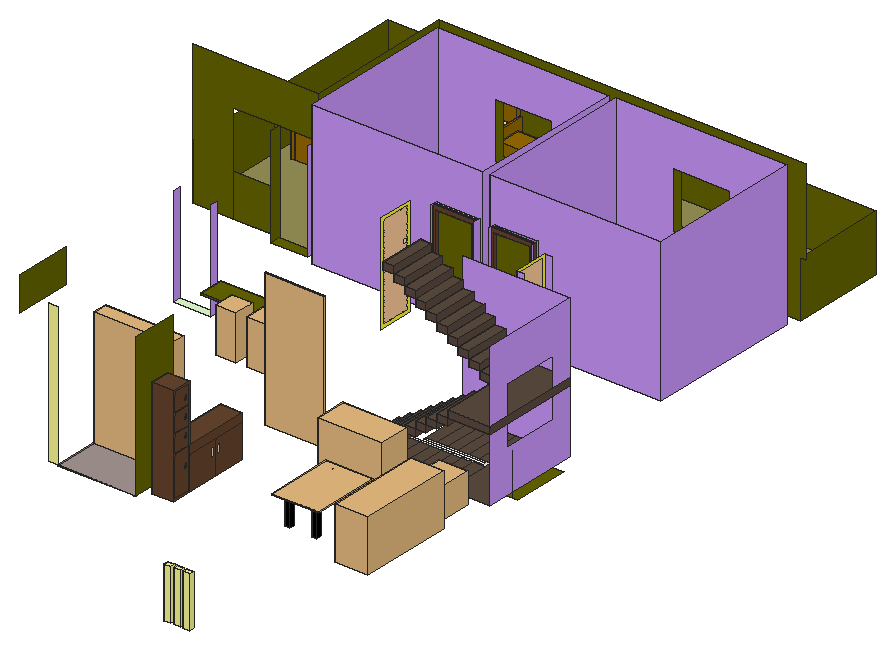
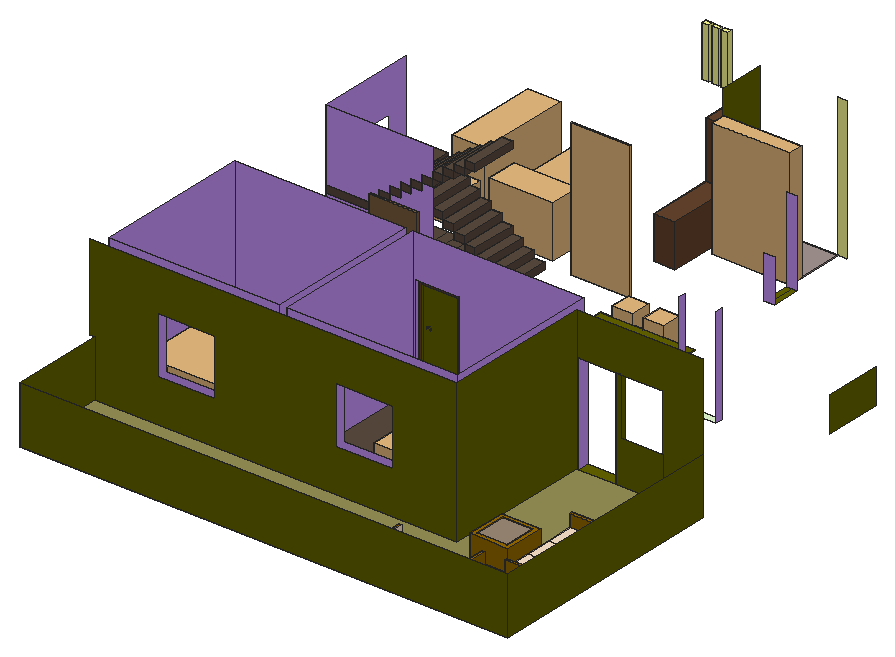
# SketchUp Ruby script. Lengths in inches.
U = 1.inch
M = Sketchup.active_model
def pt(a) = Geom::Point3d.new(a.map { |v| v * U })
def face(e, loops, mat)
  f = e.add_face(loops[0].map { |a| pt(a) })
  loops[1..].each { |l| e.add_face(l.map { |a| pt(a) }).erase! }
  f.material = f.back_material = mat if mat
  f
end
# faces: each face lists its corners as indices into pts; further lists are holes
def faces(e, pts, list, mat = nil) = list.each { |f| face(e, (f[0].is_a?(Array) ? f : [f]).map { |l| l.map { |i| pts[i] } }, mat) }
# xy, xz, yz: faces in a plane at the given z, y or x. An outline is a flat list of corners, or four numbers for a rectangle; further outlines are holes
def ring(l) = l.size == 4 ? [[l[0], l[1]], [l[2], l[1]], [l[2], l[3]], [l[0], l[3]]] : l.each_slice(2).to_a
def flat(e, list, mat, &to3) = list.each { |f| face(e, (f[0].is_a?(Array) ? f : [f]).map { |l| ring(l).map { |u, v| to3.(u, v) } }, mat) }
def xy(e, z, list, mat = nil) = flat(e, list, mat) { |x, y| [x, y, z] }
def xz(e, y, list, mat = nil) = flat(e, list, mat) { |x, z| [x, y, z] }
def yz(e, x, list, mat = nil) = flat(e, list, mat) { |y, z| [x, y, z] }
def lines(e, pts, list) = list.each { |a, b| e.add_line(pt(pts[a]), pt(pts[b])) }
# prism: a flat outline (further loops are holes) pulled along v
def prism(e, loops, v, mat = nil)
  f = face(e, loops, mat); d = Geom::Vector3d.new(v.map { |x| x * U })
  f.pushpull(f.normal.samedirection?(d) ? d.length : -d.length)
end
def box(e, o, s, mat = nil) = prism(e, [[o, [o[0] + s[0], o[1], o[2]], [o[0] + s[0], o[1] + s[1], o[2]], [o[0], o[1] + s[1], o[2]]]], [0, 0, s[2]], mat)
def at(x, y, z, deg = 0) = Geom::Transformation.translation(pt([x, y, z])) * Geom::Transformation.rotation(ORIGIN, Z_AXIS, deg.degrees)
def axes(o, x, y, z) = Geom::Transformation.new([*x, 0, *y, 0, *z, 0, *pt(o).to_a, 1])
def part(name) = M.definitions.add(name)
# library, detail: a bought-in or finely detailed component or shape, given as its bounding box
def library(name, o, s) = part(name).tap { |d| box(d.entities, o, s) }
def detail(e, o, s) = box(e.add_group.entities, o, s)
def put(e, d, t, mat = nil) = e.add_instance(d, t).tap { |i| i.material = mat if mat }
def group(e, t, mat = nil) = e.add_group.tap { |g| g.transformation = t; g.material = mat if mat }.entities
root = M.entities
M.materials.add("C01_Vanilla_Cream").color = [255, 230, 206]
M.materials.add("C02_Golden_Beige").color = [255, 205, 155]
M.materials.add("D07_Ochre_Flame").color = [153, 107, 0]
M.materials.add("E01_Mint_Frost").color = [255, 255, 204]
M.materials.add("E02_Pale_Lime").color = [255, 255, 153]
M.materials.add("E04_Green_Bloom").color = [255, 255, 49]
M.materials.add("E08_Lime_Depth").color = [102, 102, 0]
M.materials.add("Glass_Sky Reflection_01").color = [126, 138, 183]
M.materials["Glass_Sky Reflection_01"].alpha = 0.25
M.materials.add("J02_Lavender_Veil").color = [204, 153, 255]
M.materials.add("M09_Shadow_Night").color = [0, 0, 0]
M.materials.add("Marble_01_1K").color = [230, 255, 211]
M.materials.add("Marble_03_1K").color = [175, 182, 201]
M.materials.add("Marble_06_1K").color = [165, 150, 147]
M.materials.add("Marble_07_1K").color = [36, 34, 36]
M.materials.add("Marble_20_1K").color = [172, 173, 182]
M.materials.add("Metal_06_1K").color = [238, 236, 231]
M.materials.add("Plaster_02_1K").color = [157, 140, 119]
M.materials.add("Plywood_01_1K").color = [125, 96, 64]
M.materials.add("Soil_04_1K").color = [152, 146, 88]
M.materials.add("Wood_Floor_12_1K").color = [92, 75, 65]
M.materials.add("Wood_Veneer_15_1K").color = [103, 69, 45]
c1 = part("Group\#9")
box(c1.entities,[0,0,0],[0.75,3.75,0.1875],"Metal_06_1K")
c2 = part("Group\#2")
xy(c2.entities,0,[[0,-16.81,18.0625,0],[0,0,18.0625,55.25]],"Wood_Veneer_15_1K")
xy(c2.entities,36,[[0,0,18.0625,55.25]],"Wood_Veneer_15_1K")
xy(c2.entities,84,[[0,-16.81,18.0625,0]],"Wood_Veneer_15_1K")
xz(c2.entities,-16.81,[[0,0,18.0625,84]],"Wood_Veneer_15_1K")
xz(c2.entities,0,[[0,0,18.0625,36],[0,36,18.0625,84]],"Wood_Veneer_15_1K")
xz(c2.entities,55.25,[[0,0,18.0625,36]],"Wood_Veneer_15_1K")
yz(c2.entities,0,[[-16.81,0,0,84],[0,0,55.25,36]],"Wood_Veneer_15_1K")
yz(c2.entities,18.0625,[[[-16.81,0,0,84],[-14.81,2,-2,82]],[0,0,27.625,27.91],[27.625,0,55.25,27.91],[-14.81,2,-2,35],[0,27.91,55.25,36],
  [-14.81,35,-2,36],[-14.81,36,-2,50.3125],[-14.81,50.3125,-2,51.3125],[-14.81,51.3125,-2,65.85],[-14.81,65.85,-2,66.85],
  [-14.81,66.85,-2,82]],"Wood_Veneer_15_1K")
g1 = group(c2.entities,at(18.0625,23.18,16.77))
box(g1,[0,0,0],[0.2,1.5,6.25],"Metal_06_1K")
g2 = group(c2.entities,at(18.0625,29.74,16.77))
box(g2,[0,0,0],[0.2,1.5,6.25],"Metal_06_1K")
put(c2.entities,c1,axes([18.0625,-4.49,72.03],[0,1,0],[0,0,1],[1,0,0]))
put(c2.entities,c1,axes([18.0625,-4.49,57.4],[0,1,0],[0,0,1],[1,0,0]))
put(c2.entities,c1,axes([18.0625,-4.49,42.9],[0,1,0],[0,0,1],[1,0,0]))
put(c2.entities,c1,axes([18.0625,-4.49,20.71],[0,1,0],[0,0,1],[1,0,0]))
c3 = part("Group\#51")
xy(c3.entities,0,[[0,39,81,39,81,45,27,45,27,43,79,43,79,41,0,41]],"Metal_06_1K")
xy(c3.entities,0,[[0,0,9,39],[9,0,18,39],[18,0,27,39],[27,0,36,39],[36,0,45,39],
  [45,0,54,39],[54,0,63,39],[63,0,72,39],[72,0,81,39],[81,0,117,84],
  [27,45,36,84],[36,45,45,84],[45,45,54,84],[54,45,63,84],[63,45,72,84],
  [72,45,81,84]],"Wood_Floor_12_1K")
c4 = part("Group\#70")
box(c4.entities,[0,0,0],[9,39,6],"Wood_Floor_12_1K")
c5 = part("Group\#50")
xy(c5.entities,0,[[0,39,81,39,81,45,27,45,27,43,79,43,79,41,0,41]],"Metal_06_1K")
xy(c5.entities,0,[[9,0,18,39],[18,0,27,39],[27,0,36,39],[36,0,45,39],[45,0,54,39],
  [54,0,63,39],[63,0,72,39],[72,0,81,39],[81,0,117,84],[27,45,36,84],
  [36,45,45,84],[45,45,54,84],[54,45,63,84],[63,45,72,84],[72,45,81,84]],"Wood_Floor_12_1K")
put(c5.entities,c4,at(0,0,0))
put(c5.entities,c4,at(9,0,6))
put(c5.entities,c4,at(18,0,12))
put(c5.entities,c4,at(27,0,18))
put(c5.entities,c4,at(36,0,24))
put(c5.entities,c4,at(45,0,30))
put(c5.entities,c4,at(54,0,36))
put(c5.entities,c4,at(63,0,42))
put(c5.entities,c4,at(72,0,48))
g3 = group(c5.entities,at(81,0,54))
box(g3,[0,0,0],[36,84,6],"Wood_Floor_12_1K")
put(c5.entities,c4,at(72,45,60))
put(c5.entities,c4,at(63,45,66))
put(c5.entities,c4,at(54,45,72))
put(c5.entities,c4,at(45,45,78))
put(c5.entities,c4,at(36,45,84))
put(c5.entities,c4,at(27,45,90))
put(c5.entities,c4,at(18,45,96))
put(c5.entities,c4,at(9,45,102))
put(c5.entities,c4,at(0,45,108))
put(c5.entities,c4,at(-9,45,114))
c6 = part("Group\#41")
xy(c6.entities,0,[[[0,0,32.5625,34],[3.65,3.65,28.91,30.35]]],"D07_Ochre_Flame")
xy(c6.entities,18.3125,[[[0,0,32.5625,34],[3.65,3.65,28.91,30.35]]],"D07_Ochre_Flame")
xy(c6.entities,18.3125,[[3.65,3.65,28.91,30.35]],"Plaster_02_1K")
xz(c6.entities,0,[[0,0,32.5625,18.3125]],"D07_Ochre_Flame")
xz(c6.entities,3.65,[[3.65,0,28.91,18.3125]],"D07_Ochre_Flame")
xz(c6.entities,30.35,[[3.65,0,28.91,18.3125]],"D07_Ochre_Flame")
xz(c6.entities,34,[[0,0,32.5625,18.3125]],"D07_Ochre_Flame")
yz(c6.entities,0,[[0,0,34,18.3125]],"D07_Ochre_Flame")
yz(c6.entities,3.65,[[3.65,0,30.35,18.3125]],"D07_Ochre_Flame")
yz(c6.entities,28.91,[[3.65,0,30.35,18.3125]],"D07_Ochre_Flame")
yz(c6.entities,32.5625,[[0,0,34,18.3125]],"D07_Ochre_Flame")
c7 = library("Group\#27",[0,0,0],[94.3125,62.5,20])
c8 = part("Group\#17")
box(c8.entities,[0,0,0],[4,4,24])
c9 = part("Group\#16")
box(c9.entities,[0,0,0],[4,4,24])
c10 = part("Group\#29")
box(c10.entities,[0,0,0],[20.5,20.5,18],"Wood_Veneer_15_1K")
c11 = part("Group\#47")
box(c11.entities,[0,0,0],[65.6875,38.91,0.4375],"Marble_06_1K")
c12 = part("Group\#12")
detail(c12.entities,[-3,0,0],[54,27,43.625])
c13 = part("Group\#11")
detail(c13.entities,[0,0,0],[24,24,25.375])
c14 = part("Group\#10")
detail(c14.entities,[0,-4,0],[28,80,43.625])
c15 = part("Group\#14")
box(c15.entities,[0,0,0],[4,4,24])
c16 = part("Group\#15")
box(c16.entities,[0,0,0],[4,4,24])
c17 = part("Group\#38")
xy(c17.entities,0,[[67.3125,0,69.625,27.1875],[-2.33,24.1875,67.3125,27.1875]],"D07_Ochre_Flame")
xy(c17.entities,18.3125,[[0,0,22.82,24.1875],[22.82,0,45.07,24.1875],[45.07,0,67.3125,24.1875]],"C01_Vanilla_Cream")
xy(c17.entities,24.5625,[[67.3125,0,69.625,27.1875]],"D07_Ochre_Flame")
xy(c17.entities,28.6875,[[-2.33,0,0,24.1875]],"D07_Ochre_Flame")
xy(c17.entities,33.375,[[-2.33,24.1875,67.3125,27.1875]],"D07_Ochre_Flame")
xz(c17.entities,0,[[0,0,22.82,18.3125],[22.82,0,45.07,18.3125],[45.07,0,67.3125,18.3125]],"C01_Vanilla_Cream")
xz(c17.entities,0,[[-2.33,0,0,28.6875],[67.3125,0,69.625,24.5625]],"D07_Ochre_Flame")
xz(c17.entities,24.1875,[[-2.33,0,67.3125,0,67.3125,18.3125,0,18.3125,0,28.6875,-2.33,28.6875],[0,18.3125,22.82,33.375],[22.82,18.3125,45.07,33.375],[45.07,18.3125,67.3125,33.375],[-2.33,28.6875,0,33.375]],"D07_Ochre_Flame")
xz(c17.entities,27.1875,[[-2.33,0,67.3125,33.375],[67.3125,0,69.625,24.5625]],"D07_Ochre_Flame")
yz(c17.entities,-2.33,[[0,0,24.1875,28.6875],[24.1875,0,27.1875,33.375]],"D07_Ochre_Flame")
yz(c17.entities,0,[[0,18.3125,24.1875,28.6875]],"D07_Ochre_Flame")
yz(c17.entities,67.3125,[[0,0,24.1875,18.3125],[0,18.3125,24.1875,24.5625]],"C01_Vanilla_Cream")
yz(c17.entities,67.3125,[[24.1875,0,27.1875,24.5625],[24.1875,24.5625,27.1875,33.375]],"D07_Ochre_Flame")
yz(c17.entities,69.625,[[0,0,27.1875,24.5625]],"D07_Ochre_Flame")
c18 = part("Group\#43")
box(c18.entities,[0,0,0],[1,4.5625,0.25],"Metal_06_1K")
c19 = part("Group\#42")
xy(c19.entities,0,[[0,-1.93,40.35,0],[0,0,40.35,21.25]],"Plywood_01_1K")
xy(c19.entities,25.125,[[0,0,40.35,21.25]],"Marble_07_1K")
xy(c19.entities,25.1875,[[20.85,8.75,21.39,8.86,21.89,9.11,22.3,9.47,22.61,9.94,22.79,10.46,22.82,11.01,22.71,11.56,22.47,12.06,22.1,12.47,21.64,12.78,21.11,12.96,20.56,12.99,20.01,12.88,19.52,12.63,19.1,12.27,18.79,11.81,18.62,11.28,18.58,10.73,18.69,10.18,18.9375,9.69,19.31,9.27,19.77,8.96,20.29,8.79]],"M09_Shadow_Night")
xy(c19.entities,25.1875,[[[8.8,4,31.8,17.68],[20.85,8.75,20.29,8.79,19.77,8.96,19.31,9.27,18.9375,9.69,18.69,10.18,18.58,10.73,18.62,11.28,18.79,11.81,19.1,12.27,19.52,12.63,20.01,12.88,20.56,12.99,21.11,12.96,21.64,12.78,22.1,12.47,22.47,12.06,22.71,11.56,22.82,11.01,22.79,10.46,22.61,9.94,22.3,9.47,21.89,9.11,21.39,8.86]]],"Marble_07_1K")
xy(c19.entities,26,[[0,-1.93,40.35,0]],"Plywood_01_1K")
xy(c19.entities,26.5625,[[[0,0,40.35,21.25],[8.8,4,31.8,17.68]]],"Marble_07_1K")
xy(c19.entities,71.66,[[0,-1.93,40.35,0]],"Plywood_01_1K")
xz(c19.entities,-1.93,[[0,0,40.35,26],[0,26,40.35,71.66]],"Plywood_01_1K")
xz(c19.entities,0,[[0,25.125,40.35,26],[0,26,40.35,26.5625]],"Marble_07_1K")
xz(c19.entities,0,[[0,0,40.35,25.125],[0,26.5625,40.35,71.66]],"Plywood_01_1K")
xz(c19.entities,4,[[8.8,25.1875,31.8,26.5625]],"Marble_07_1K")
xz(c19.entities,17.68,[[8.8,25.1875,31.8,26.5625]],"Marble_07_1K")
xz(c19.entities,21.25,[[0,25.125,40.35,26.5625]],"Marble_07_1K")
xz(c19.entities,21.25,[[0,0,20.17,21],[20.17,0,40.35,21],[0,21,40.35,25.125]],"Plywood_01_1K")
yz(c19.entities,0,[[0,25.125,21.25,26.5625]],"Marble_07_1K")
yz(c19.entities,0,[[-1.93,0,0,26],[0,0,21.25,25.125],[-1.93,26,0,71.66]],"Plywood_01_1K")
yz(c19.entities,8.8,[[4,25.1875,17.68,26.5625]],"Marble_07_1K")
yz(c19.entities,31.8,[[4,25.1875,17.68,26.5625]],"Marble_07_1K")
yz(c19.entities,40.35,[[0,25.125,21.25,26.5625]],"Marble_07_1K")
yz(c19.entities,40.35,[[-1.93,0,0,26],[0,0,21.25,25.125],[-1.93,26,0,71.66]],"Plywood_01_1K")
put(c19.entities,c18,axes([22.63,21.25,13.17],[-1,0,0],[0,0,1],[0,1,0]))
put(c19.entities,c18,axes([18.69,21.25,13.17],[-1,0,0],[0,0,1],[0,1,0]))
put(c19.entities,c18,axes([22.61,21.25,24.2],[0,0,-1],[-1,0,0],[0,1,0]))
c20 = part("Group\#40")
box(c20.entities,[0,4,0],[19.9375,19.25,18.3125],"D07_Ochre_Flame")
c21 = library("Group\#36",[0,0,0],[17.25,17.25,38])
c22 = library("Group\#54",[0,-12,0],[65.6875,12,119.5625])
c23 = part("Group\#61")
prism(c23.entities,[[[0.51,0.51,0],[0.23,0.875,0],[0.06,1.3,0],[0,1.75,0],[0.06,2.2,0],[0.23,2.625,0],[0.51,2.99,0],[0.875,3.27,0],[1.3,3.44,0],[1.75,3.5,0],[2.2,3.44,0],[2.625,3.27,0],[2.99,2.99,0],[3.27,2.625,0],[3.44,2.2,0],[3.5,1.75,0],[3.44,1.3,0],[3.27,0.875,0],[2.99,0.51,0],[2.625,0.23,0],[2.2,0.06,0],[1.75,0,0],[1.3,0.06,0],[0.875,0.23,0]]],[0,0,0.625],"Metal_06_1K")
c24 = part("Group\#59")
xy(c24.entities,0,[[0,-2,36,0]],"Wood_Veneer_15_1K")
xy(c24.entities,3,[[3,-0.5,33,0]])
xy(c24.entities,3,[[3,-2,33,-0.5]],"Wood_Veneer_15_1K")
xy(c24.entities,81,[[3,-0.5,33,0]])
xy(c24.entities,81,[[3,-2,33,-0.5]],"Wood_Veneer_15_1K")
xy(c24.entities,84,[[0,-2,36,0]],"Wood_Veneer_15_1K")
xz(c24.entities,-2,[[[0,0,36,84],[3,3,33,81]]],"Wood_Veneer_15_1K")
xz(c24.entities,-0.5,[[3,3,33,81]])
xz(c24.entities,0,[[[0,0,36,84],[3,3,33,81]]],"Wood_Veneer_15_1K")
yz(c24.entities,0,[[-2,0,0,84]],"Wood_Veneer_15_1K")
yz(c24.entities,3,[[-0.5,3,0,81]])
yz(c24.entities,3,[[-2,3,-0.5,81]],"Wood_Veneer_15_1K")
yz(c24.entities,33,[[-0.5,3,0,81]])
yz(c24.entities,33,[[-2,3,-0.5,81]],"Wood_Veneer_15_1K")
yz(c24.entities,36,[[-2,0,0,84]],"Wood_Veneer_15_1K")
put(c24.entities,c23,axes([25.79,-0.5,47.4],[1,0,0],[0,0,1],[0,-1,0]))
put(c24.entities,c23,axes([57.22,-0.5,47.4],[1,0,0],[0,0,1],[0,-1,0]))
c25 = part("Group\#60")
xy(c25.entities,0,[[0,-2,36,0]],"Wood_Veneer_15_1K")
xy(c25.entities,3,[[3,-0.5,33,0]])
xy(c25.entities,3,[[3,-2,33,-0.5]],"Wood_Veneer_15_1K")
xy(c25.entities,81,[[3,-0.5,33,0]])
xy(c25.entities,81,[[3,-2,33,-0.5]],"Wood_Veneer_15_1K")
xy(c25.entities,84,[[0,-2,36,0]],"Wood_Veneer_15_1K")
xz(c25.entities,-2,[[[0,0,36,84],[3,3,33,81]]],"Wood_Veneer_15_1K")
xz(c25.entities,-0.5,[[3,3,33,81]])
xz(c25.entities,0,[[[0,0,36,84],[3,3,33,81]]],"Wood_Veneer_15_1K")
yz(c25.entities,0,[[-2,0,0,84]],"Wood_Veneer_15_1K")
yz(c25.entities,3,[[-0.5,3,0,81]])
yz(c25.entities,3,[[-2,3,-0.5,81]],"Wood_Veneer_15_1K")
yz(c25.entities,33,[[-0.5,3,0,81]])
yz(c25.entities,33,[[-2,3,-0.5,81]],"Wood_Veneer_15_1K")
yz(c25.entities,36,[[-2,0,0,84]],"Wood_Veneer_15_1K")
c26 = part("Group\#62")
yz(c26.entities,-0.625,[[5.65,55.09,5.28,55.14,4.93,55.28,4.64,55.51,4.41,55.81,4.26,56.15,4.22,56.53,4.26,56.9,4.41,57.25,4.64,57.54,4.93,57.77,5.28,57.92,5.65,57.96,6.03,57.92,6.37,57.77,6.67,57.54,6.9,57.25,7.04,56.9,7.09,56.53,7.04,56.15,6.9,55.81,6.67,55.51,6.37,55.28,6.03,55.14]],"Metal_06_1K")
yz(c26.entities,0,[[[2.8125,2.8125,27.1875,81.1875],[5.65,55.09,6.03,55.14,6.37,55.28,6.67,55.51,6.9,55.81,7.04,56.15,7.09,56.53,7.04,56.9,6.9,57.25,6.67,57.54,6.37,57.77,6.03,57.92,5.65,57.96,5.28,57.92,4.93,57.77,4.64,57.54,4.41,57.25,4.26,56.9,4.22,56.53,4.26,56.15,4.41,55.81,4.64,55.51,4.93,55.28,5.28,55.14]]],"C02_Golden_Beige")
yz(c26.entities,0,[[[0,0,30,84],[2.8125,2.8125,27.1875,81.1875]]],"E04_Green_Bloom")
p = [[0,5.28,55.14],[0,4.93,55.28],[-0.625,4.93,55.28],[-0.625,5.28,55.14],[0,5.65,55.09],[-0.625,5.65,55.09],
  [0,6.03,55.14],[-0.625,6.03,55.14],[0,6.37,55.28],[-0.625,6.37,55.28],[0,4.64,55.51],[-0.625,4.64,55.51],
  [0,6.67,55.51],[-0.625,6.67,55.51],[0,4.41,55.81],[-0.625,4.41,55.81],[0,6.9,55.81],[-0.625,6.9,55.81],
  [0,4.26,56.15],[-0.625,4.26,56.15],[0,7.04,56.15],[-0.625,7.04,56.15],[0,4.22,56.53],[-0.625,4.22,56.53],
  [0,7.09,56.53],[-0.625,7.09,56.53],[0,4.26,56.9],[-0.625,4.26,56.9],[0,7.04,56.9],[-0.625,7.04,56.9],
  [0,4.41,57.25],[-0.625,4.41,57.25],[0,6.9,57.25],[-0.625,6.9,57.25],[0,4.64,57.54],[-0.625,4.64,57.54],
  [0,6.67,57.54],[-0.625,6.67,57.54],[0,4.93,57.77],[-0.625,4.93,57.77],[0,6.37,57.77],[-0.625,6.37,57.77],
  [0,5.28,57.92],[-0.625,5.28,57.92],[0,6.03,57.92],[-0.625,6.03,57.92],[0,5.65,57.96],[-0.625,5.65,57.96]]
faces(c26.entities,p,[[0,1,2,3],[4,0,3,5],[6,4,5,7],[8,6,7,9],[1,10,11,2],[12,8,9,13],[10,14,15,11],[16,12,13,17],
  [14,18,19,15],[20,16,17,21],[18,22,23,19],[24,20,21,25],[22,26,27,23],[28,24,25,29],[26,30,31,27],[32,28,29,33],
  [30,34,35,31],[36,32,33,37],[34,38,39,35],[40,36,37,41],[38,42,43,39],[44,40,41,45],[42,46,47,43],[46,44,45,47]],"Metal_06_1K")
c27 = library("Group\#63",[-3.99,-1.7,0],[49.63,1.7,114.25])
c28 = library("Group\#28",[0,0,0],[94.3125,62.5,20])
c29 = part("Group\#74")
box(c29.entities,[0,-4,0],[5.875,4,42.75],"E02_Pale_Lime")
c30 = part("Group\#13")
detail(c30.entities,[-5.9375,-5.9375,0],[39.25,56.8125,1])
xy(root,174,[[1713.42,1916.04,1717.92,1940.04],[1717.92,1916.04,1722.42,1940.04],[1978.04,2015.58,1987.04,2063.58],[1761.26,2060.28,1763.8,2081.58],[1644.54,2183.58,1675.875,2192.58]],"E08_Lime_Depth")
xy(root,174,[[1644.54,2081.58,1675.875,2087.58]],"Marble_01_1K")
xy(root,174,[[1888.04,2137.61,1894.04,2167.61]],"Marble_03_1K")
xy(root,174,[[1722.42,1862.58,1788.11,1901.49]],"Marble_20_1K")
xy(root,174,[[1571.73,2192.58,1678.04,2192.58,1678.04,2318.58,1982.36,2318.58,1982.36,2397.95,1571.73,2397.95]],"Soil_04_1K")
xy(root,174,[[1684.04,2177.58,1828.04,2309.58],[1834.04,2177.58,1978.04,2309.58]],"Wood_Floor_12_1K")
xy(root,174,[[1788.97,2171.58,1824.97,2177.58],[1837.82,2171.58,1873.82,2177.58]],"Wood_Veneer_15_1K")
xy(root,202.6875,[[1684.04,2060.28,1761.26,2081.58],[1761.26,2060.28,1763.8,2081.58]],"E08_Lime_Depth")
xy(root,203.6875,[[1684.04,2060.28,1763.8,2081.58]],"E08_Lime_Depth")
xz(root,1862.58,[[1714.42,174.4375,1722.42,294]],"E02_Pale_Lime")
xz(root,1916.04,[[1713.42,174,1722.42,246]],"J02_Lavender_Veil")
xz(root,1940.04,[[1713.42,174,1722.42,210]],"J02_Lavender_Veil")
xz(root,2060.28,[[1761.26,174,1763.8,202.6875],[1684.04,202.6875,1763.8,203.6875]],"E08_Lime_Depth")
xz(root,2081.58,[[1761.26,174,1763.8,202.6875],[1684.04,202.6875,1763.8,203.6875]],"E08_Lime_Depth")
xz(root,2081.58,[[1888.04,174,1978.04,294]],"J02_Lavender_Veil")
xz(root,2137.61,[[1888.04,174,1894.04,258]],"J02_Lavender_Veil")
xz(root,2167.61,[[1888.04,174,1894.04,258]],"J02_Lavender_Veil")
xz(root,2177.58,[[1684.04,174,1684.04,294,1828.04,294,1828.04,174,1824.97,174,1824.97,258,1788.97,258,1788.97,174],[1834.04,174,1834.04,294,1978.04,294,1978.04,174,1873.82,174,1873.82,258,1837.82,258,1837.82,174]],"J02_Lavender_Veil")
xz(root,2192.58,[[1571.73,174,1571.73,294,1678.04,294,1678.04,174,1675.875,174,1675.875,258,1644.54,258,1644.54,258.0625,1641.14,258.0625,1641.14,258,1605.14,258,1605.14,174],[1605.14,174,1605.14,210,1641.14,210,1641.14,258,1644.54,258,1644.54,174]],"E08_Lime_Depth")
xz(root,2309.58,[[[1684.04,174,1828.04,294],[1732.04,210,1780.04,258]],[[1834.04,174,1978.04,294],[1882.04,210,1930.04,258]]],"J02_Lavender_Veil")
xz(root,2318.58,[[[1678.04,174,1678.04,294,1987.04,294,1987.04,222,1982.36,222,1982.36,174],[1882.04,210,1930.04,258],[1732.04,210,1780.04,258]]],"E08_Lime_Depth")
xz(root,2397.95,[[1571.73,174,1982.36,222]],"E08_Lime_Depth")
yz(root,1571.73,[[2192.58,174,2397.95,222]],"E08_Lime_Depth")
yz(root,1576.04,[[2005.11,175,2053.11,204]],"E08_Lime_Depth")
yz(root,1644.54,[[2183.58,174,2192.58,258.0625]],"E08_Lime_Depth")
yz(root,1644.54,[[2081.58,174,2087.58,258]],"J02_Lavender_Veil")
yz(root,1675.875,[[2081.58,174,2087.58,258],[2183.58,174,2192.58,258]],"J02_Lavender_Veil")
yz(root,1678.04,[[2192.58,174,2318.58,294]],"E08_Lime_Depth")
yz(root,1684.04,[[2060.28,202.6875,2081.58,203.6875]],"E08_Lime_Depth")
yz(root,1684.04,[[2177.58,174,2309.58,294]],"J02_Lavender_Veil")
yz(root,1761.26,[[2060.28,174,2081.58,202.6875]],"E08_Lime_Depth")
yz(root,1763.8,[[2060.28,174,2081.58,202.6875],[2060.28,202.6875,2081.58,203.6875]],"E08_Lime_Depth")
yz(root,1788.11,[[1862.58,174,1901.49,294]],"E08_Lime_Depth")
yz(root,1788.97,[[2171.58,174,2177.58,258]],"J02_Lavender_Veil")
yz(root,1824.97,[[2171.58,174,2177.58,258]],"J02_Lavender_Veil")
yz(root,1828.04,[[2177.58,174,2309.58,294]],"J02_Lavender_Veil")
yz(root,1834.04,[[2177.58,174,2309.58,294]],"J02_Lavender_Veil")
yz(root,1837.82,[[2171.58,174,2177.58,258]],"J02_Lavender_Veil")
yz(root,1873.82,[[2171.58,174,2177.58,258]],"J02_Lavender_Veil")
yz(root,1978.04,[[[1997.58,174,2081.58,294],[2015.58,210,2063.58,258]],[2177.58,174,2309.58,294]],"J02_Lavender_Veil")
yz(root,1982.36,[[2318.58,174,2397.95,222]],"E08_Lime_Depth")
p = [[1982.54,2015.58,174],[1982.54,2015.58,210]]
lines(root,p,[[0,1]])
put(root,c2,at(1794.11,1888.38,174),"E08_Lime_Depth")
put(root,c3,at(1861.04,1997.58,174),"E08_Lime_Depth")
put(root,c5,at(1861.04,1997.58,174),"E08_Lime_Depth")
put(root,c6,at(1625.93,2295.69,174),"E08_Lime_Depth")
put(root,c7,at(1973.14,2280.46,174,-180),"E08_Lime_Depth")
put(root,c8,at(1912.35,1934.16,174),"M09_Shadow_Night")
put(root,c9,at(1889.29,1934.16,174),"M09_Shadow_Night")
put(root,c10,at(1952.64,2280.46,174),"E01_Mint_Frost")
put(root,c11,at(1722.42,1862.58,174),"E08_Lime_Depth")
put(root,c10,at(1952.64,2197.46,174),"E01_Mint_Frost")
put(root,c12,at(1867.15,1958.1875,174),"E08_Lime_Depth")
put(root,c13,at(1941.19,1965.86,174),"E08_Lime_Depth")
put(root,c14,at(1945.27,1879.05,174),"E08_Lime_Depth")
put(root,c15,at(1889.29,1892.47,174),"M09_Shadow_Night")
put(root,c16,at(1912.35,1892.47,174),"M09_Shadow_Night")
put(root,c17,at(1611.81,2282.16,174,90.739),"E08_Lime_Depth")
put(root,c19,at(1894.64,2089.5,174),"E08_Lime_Depth")
put(root,c17,at(1625.98,2357.15,174),"E08_Lime_Depth")
put(root,c20,at(1698.42,2353.12,174),"D07_Ochre_Flame")
put(root,c21,at(1710.39,2043.07,174),"E08_Lime_Depth")
put(root,c21,at(1736.76,2043.07,174),"E08_Lime_Depth")
put(root,c22,axes([1722.42,1912.1875,174],[1,0,0],[0,1,0],[0,0,0.83]),"Wood_Veneer_15_1K")
put(root,c24,at(1788.97,2175.33,174),"E08_Lime_Depth")
put(root,c25,at(1837.82,2175.33,174),"E08_Lime_Depth")
put(root,c26,at(1888.04,2137.61,174),"E08_Lime_Depth")
put(root,c26,at(1774.04,2167.61,174,-180),"E08_Lime_Depth")
put(root,c27,at(1798.09,1991.58,174),"E02_Pale_Lime")
put(root,c10,at(1687.15,2193.61,174),"E01_Mint_Frost")
put(root,c28,at(1687.15,2214.11,174),"E08_Lime_Depth")
put(root,c10,at(1687.15,2276.61,174),"E01_Mint_Frost")
put(root,c29,at(1928.34,1740.42,179.25))
put(root,c29,at(1920.34,1740.42,179.25))
put(root,c29,at(1912.34,1740.42,179.25))
put(root,c30,at(1889.29,1892.47,198),"Glass_Sky Reflection_01")
